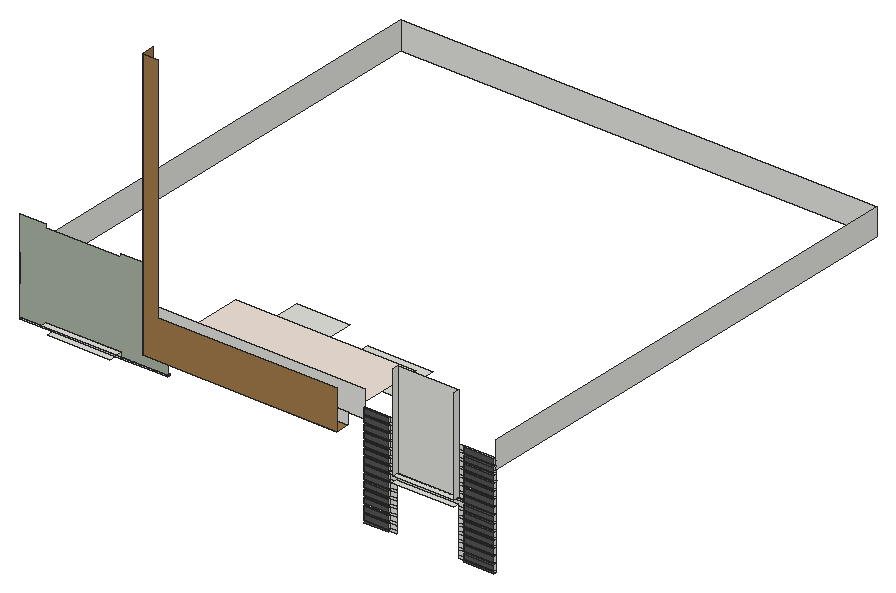
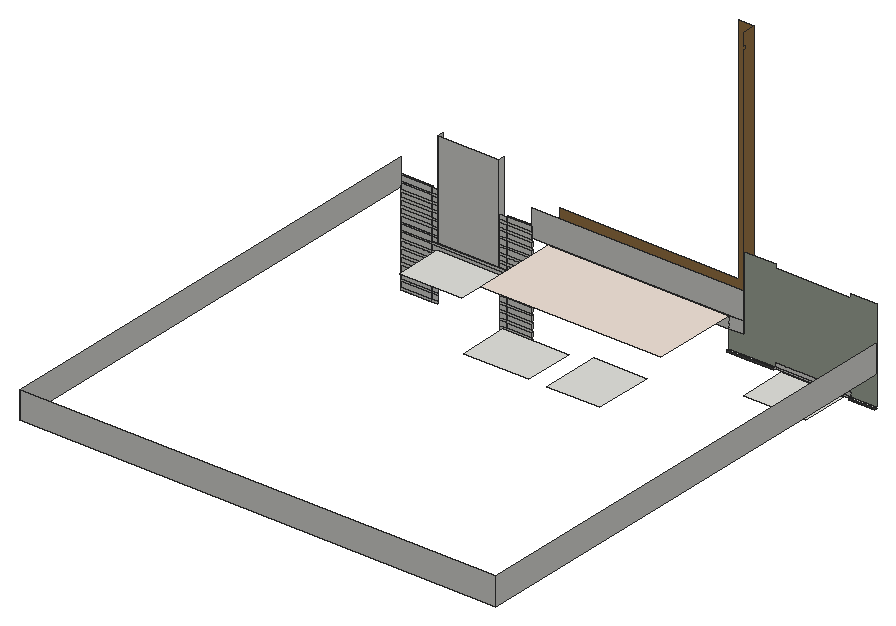
# SketchUp Ruby script. Lengths in inches.
U = 1.inch
M = Sketchup.active_model
def pt(a) = Geom::Point3d.new(a.map { |v| v * U })
def face(e, loops, mat)
  f = e.add_face(loops[0].map { |a| pt(a) })
  loops[1..].each { |l| e.add_face(l.map { |a| pt(a) }).erase! }
  f.material = f.back_material = mat if mat
  f
end
# faces: each face lists its corners as indices into pts; further lists are holes
def faces(e, pts, list, mat = nil) = list.each { |f| face(e, (f[0].is_a?(Array) ? f : [f]).map { |l| l.map { |i| pts[i] } }, mat) }
# xy, xz, yz: faces in a plane at the given z, y or x. An outline is a flat list of corners, or four numbers for a rectangle; further outlines are holes
def ring(l) = l.size == 4 ? [[l[0], l[1]], [l[2], l[1]], [l[2], l[3]], [l[0], l[3]]] : l.each_slice(2).to_a
def flat(e, list, mat, &to3) = list.each { |f| face(e, (f[0].is_a?(Array) ? f : [f]).map { |l| ring(l).map { |u, v| to3.(u, v) } }, mat) }
def xy(e, z, list, mat = nil) = flat(e, list, mat) { |x, y| [x, y, z] }
def xz(e, y, list, mat = nil) = flat(e, list, mat) { |x, z| [x, y, z] }
def yz(e, x, list, mat = nil) = flat(e, list, mat) { |y, z| [x, y, z] }
def lines(e, pts, list) = list.each { |a, b| e.add_line(pt(pts[a]), pt(pts[b])) }
# prism: a flat outline (further loops are holes) pulled along v
def prism(e, loops, v, mat = nil)
  f = face(e, loops, mat); d = Geom::Vector3d.new(v.map { |x| x * U })
  f.pushpull(f.normal.samedirection?(d) ? d.length : -d.length)
end
def box(e, o, s, mat = nil) = prism(e, [[o, [o[0] + s[0], o[1], o[2]], [o[0] + s[0], o[1] + s[1], o[2]], [o[0], o[1] + s[1], o[2]]]], [0, 0, s[2]], mat)
def at(x, y, z, deg = 0) = Geom::Transformation.translation(pt([x, y, z])) * Geom::Transformation.rotation(ORIGIN, Z_AXIS, deg.degrees)
def axes(o, x, y, z) = Geom::Transformation.new([*x, 0, *y, 0, *z, 0, *pt(o).to_a, 1])
def part(name) = M.definitions.add(name)
# library, detail: a bought-in or finely detailed component or shape, given as its bounding box
def library(name, o, s) = part(name).tap { |d| box(d.entities, o, s) }
def detail(e, o, s) = box(e.add_group.entities, o, s)
def put(e, d, t, mat = nil) = e.add_instance(d, t).tap { |i| i.material = mat if mat }
def group(e, t, mat = nil) = e.add_group.tap { |g| g.transformation = t; g.material = mat if mat }.entities
root = M.entities
M.materials.add("Generic\#1").color = [85, 85, 85]
M.materials.add("Generic\#2").color = [170, 178, 163]
M.materials.add("Generic\#3").color = [162, 123, 74]
M.materials.add("Generic\#4").color = [241, 227, 216]
xy(root,660.3125,[[395.4375,28.5,423.8125,31.0625],[508.98,28.5,543.6875,31.0625]],"Generic\#1")
xy(root,663.125,[[395.4375,28.5,423.8125,31.0625],[508.98,28.5,543.6875,31.0625]],"Generic\#1")
xy(root,668.625,[[395.4375,28.5,423.8125,31.0625],[508.98,28.5,543.6875,31.0625]],"Generic\#1")
xy(root,671.4375,[[395.4375,28.5,423.8125,31.0625],[508.98,28.5,543.6875,31.0625]],"Generic\#1")
xy(root,676.9375,[[395.4375,28.5,423.8125,31.0625],[508.98,28.5,543.6875,31.0625]],"Generic\#1")
xy(root,679.75,[[395.4375,28.5,423.8125,31.0625],[508.98,28.5,543.6875,31.0625]],"Generic\#1")
xy(root,685.25,[[395.4375,28.5,423.8125,31.0625],[508.98,28.5,543.6875,31.0625]],"Generic\#1")
xy(root,688.0625,[[395.4375,28.5,423.8125,31.0625],[508.98,28.5,543.6875,31.0625]],"Generic\#1")
xy(root,693.5625,[[395.4375,28.5,423.8125,31.0625],[508.98,28.5,543.6875,31.0625]],"Generic\#1")
xy(root,696.375,[[395.4375,28.5,423.8125,31.0625],[508.98,28.5,543.6875,31.0625]],"Generic\#1")
xy(root,701.875,[[395.4375,28.5,423.8125,31.0625],[508.98,28.5,543.6875,31.0625]],"Generic\#1")
xy(root,704.6875,[[395.4375,28.5,423.8125,31.0625],[508.98,28.5,543.6875,31.0625]],"Generic\#1")
xy(root,710.1875,[[395.4375,28.5,423.8125,31.0625],[508.98,28.5,543.6875,31.0625]],"Generic\#1")
xy(root,713,[[395.4375,28.5,423.8125,31.0625],[508.98,28.5,543.6875,31.0625]],"Generic\#1")
xy(root,715.02,[[430.99,24.0625,501.8,31.0625],[430.99,31.0625,501.8,85.4375]])
xy(root,718.5,[[395.4375,28.5,423.8125,31.0625],[508.98,28.5,543.6875,31.0625]],"Generic\#1")
xy(root,721.3125,[[395.4375,28.5,423.8125,31.0625],[508.98,28.5,543.6875,31.0625]],"Generic\#1")
xy(root,722.19,[[431.91,24.0625,501.98,31.0625]])
xy(root,726.8125,[[395.4375,28.5,423.8125,31.0625],[508.98,28.5,543.6875,31.0625]],"Generic\#1")
xy(root,728.2,[[40.36,24.0625,111.18,31.0625],[40.36,31.0625,111.18,85.4375]])
xy(root,728.625,[[3.6875,31.0625,33.1875,32.9375],[118.35,31.0625,154.5,32.9375],[154.5,31.0625,171.6875,32.9375]])
xy(root,729.625,[[395.4375,28.5,423.8125,31.0625],[508.98,28.5,543.6875,31.0625]],"Generic\#1")
xy(root,730.04,[[275.98,127,350.54,183.625]])
xy(root,730.625,[[3.6875,31.0625,33.1875,32.9375],[118.35,31.0625,154.5,32.9375],[154.5,31.0625,171.6875,32.9375]])
xy(root,735.125,[[395.4375,28.5,423.8125,31.0625],[508.98,28.5,543.6875,31.0625]],"Generic\#1")
xy(root,735.38,[[33.1875,24.0625,118.35,31.0625]])
xy(root,737.0625,[[187.38,127,247.51,193.75]])
xy(root,737.9375,[[395.4375,28.5,423.8125,31.0625],[508.98,28.5,543.6875,31.0625]],"Generic\#1")
xy(root,743.4375,[[395.4375,28.5,423.8125,31.0625],[508.98,28.5,543.6875,31.0625]],"Generic\#1")
xy(root,746.25,[[395.4375,28.5,423.8125,31.0625],[508.98,28.5,543.6875,31.0625]],"Generic\#1")
xy(root,751.4375,[[154.5,15.8125,375.6875,31.0625]],"Generic\#3")
xy(root,751.75,[[395.4375,28.5,423.8125,31.0625],[508.98,28.5,543.6875,31.0625]],"Generic\#1")
xy(root,754.5625,[[395.4375,28.5,423.8125,31.0625],[508.98,28.5,543.6875,31.0625]],"Generic\#1")
xy(root,760.0625,[[395.4375,28.5,423.8125,31.0625],[508.98,28.5,543.6875,31.0625]],"Generic\#1")
xy(root,762.875,[[395.4375,28.5,423.8125,31.0625],[508.98,28.5,543.6875,31.0625]],"Generic\#1")
xy(root,764.625,[[171.6875,31.0625,375.6875,127]],"Generic\#4")
xy(root,768.375,[[395.4375,28.5,423.8125,31.0625],[508.98,28.5,543.6875,31.0625]],"Generic\#1")
xy(root,771.1875,[[395.4375,28.5,423.8125,31.0625],[508.98,28.5,543.6875,31.0625]],"Generic\#1")
xz(root,15.8125,[[154.5,751.4375,375.6875,751.4375,375.6875,795.5,171.6875,795.5,171.6875,1058.1875,154.5,1058.1875]],"Generic\#3")
xz(root,28.5,[[395.4375,663.125,423.8125,668.625],[508.98,663.125,543.6875,668.625],[395.4375,671.4375,423.8125,676.9375],[508.98,671.4375,543.6875,676.9375],[395.4375,679.75,423.8125,685.25],
  [508.98,679.75,543.6875,685.25],[395.4375,688.0625,423.8125,693.5625],[508.98,688.0625,543.6875,693.5625],[395.4375,696.375,423.8125,701.875],[508.98,696.375,543.6875,701.875],
  [395.4375,704.6875,423.8125,710.1875],[508.98,704.6875,543.6875,710.1875],[395.4375,713,423.8125,718.5],[508.98,713,543.6875,718.5],[395.4375,721.3125,423.8125,726.8125],
  [508.98,721.3125,543.6875,726.8125],[395.4375,729.625,423.8125,735.125],[508.98,729.625,543.6875,735.125],[395.4375,737.9375,423.8125,743.4375],[508.98,737.9375,543.6875,743.4375],
  [395.4375,746.25,423.8125,751.75],[508.98,746.25,543.6875,751.75],[395.4375,754.5625,423.8125,760.0625],[508.98,754.5625,543.6875,760.0625],[395.4375,762.875,423.8125,768.375],
  [508.98,762.875,543.6875,768.375],[395.4375,771.1875,423.8125,776.6875],[508.98,771.1875,543.6875,776.6875]],"Generic\#1")
xz(root,31.0625,[[395.4375,660.3125,423.8125,663.125],[423.8125,660.3125,430.99,663.125],[501.8,660.3125,508.98,663.125],[508.98,660.3125,543.6875,663.125],[395.4375,663.125,423.8125,668.625],
  [423.8125,663.125,430.99,668.625],[501.8,663.125,508.98,668.625],[508.98,663.125,543.6875,668.625],[395.4375,668.625,423.8125,671.4375],[423.8125,668.625,430.99,671.4375],
  [501.8,668.625,508.98,671.4375],[508.98,668.625,543.6875,671.4375],[395.4375,671.4375,423.8125,676.9375],[423.8125,671.4375,430.99,676.9375],[501.8,671.4375,508.98,676.9375],
  [508.98,671.4375,543.6875,676.9375],[395.4375,676.9375,423.8125,679.75],[423.8125,676.9375,430.99,679.75],[501.8,676.9375,508.98,679.75],[508.98,676.9375,543.6875,679.75],
  [395.4375,679.75,423.8125,685.25],[423.8125,679.75,430.99,685.25],[501.8,679.75,508.98,685.25],[508.98,679.75,543.6875,685.25],[395.4375,685.25,423.8125,688.0625],
  [423.8125,685.25,430.99,688.0625],[501.8,685.25,508.98,688.0625],[508.98,685.25,543.6875,688.0625],[395.4375,688.0625,423.8125,693.5625],[423.8125,688.0625,430.99,693.5625],
  [501.8,688.0625,508.98,693.5625],[508.98,688.0625,543.6875,693.5625],[395.4375,693.5625,423.8125,696.375],[423.8125,693.5625,430.99,696.375],[501.8,693.5625,508.98,696.375],
  [508.98,693.5625,543.6875,696.375],[395.4375,696.375,423.8125,701.875],[423.8125,696.375,430.99,701.875],[501.8,696.375,508.98,701.875],[508.98,696.375,543.6875,701.875],
  [395.4375,701.875,423.8125,704.6875],[423.8125,701.875,430.99,704.6875],[501.8,701.875,508.98,704.6875],[508.98,701.875,543.6875,704.6875],[395.4375,704.6875,423.8125,710.1875],
  [423.8125,704.6875,430.99,710.1875],[501.8,704.6875,508.98,710.1875],[508.98,704.6875,543.6875,710.1875],[395.4375,710.1875,423.8125,713],[423.8125,710.1875,430.99,713],
  [501.8,710.1875,508.98,713],[508.98,710.1875,543.6875,713],[395.4375,713,423.8125,718.5],[423.8125,713,430.99,713,430.99,715.02,501.8,715.02,501.8,713,508.98,713,508.98,718.5,423.8125,718.5],[508.98,713,543.6875,718.5],
  [395.4375,718.5,423.8125,721.3125],[423.8125,718.5,508.98,721.3125],[508.98,718.5,543.6875,721.3125],[395.4375,721.3125,423.8125,726.8125],[423.8125,721.3125,508.98,722.19],
  [508.98,721.3125,543.6875,726.8125],[423.8125,722.19,431.91,726.8125],[431.91,722.19,501.98,831.53],[501.98,722.19,508.98,726.8125],[395.4375,726.8125,423.8125,729.625],
  [423.8125,726.8125,431.91,729.625],[501.98,726.8125,508.98,729.625],[508.98,726.8125,543.6875,729.625],[33.1875,728.625,118.35,730.625],[395.4375,729.625,423.8125,735.125],
  [423.8125,729.625,431.91,735.125],[501.98,729.625,508.98,735.125],[508.98,729.625,543.6875,735.125],[33.1875,730.625,118.35,735.38],[395.4375,735.125,423.8125,737.9375],
  [423.8125,735.125,431.91,737.9375],[501.98,735.125,508.98,737.9375],[508.98,735.125,543.6875,737.9375],[395.4375,737.9375,423.8125,743.4375],[423.8125,737.9375,431.91,743.4375],
  [501.98,737.9375,508.98,743.4375],[508.98,737.9375,543.6875,743.4375],[395.4375,743.4375,423.8125,746.25],[423.8125,743.4375,431.91,746.25],[501.98,743.4375,508.98,746.25],
  [508.98,743.4375,543.6875,746.25],[395.4375,746.25,423.8125,751.75],[423.8125,746.25,431.91,751.75],[501.98,746.25,508.98,751.75],[508.98,746.25,543.6875,751.75],
  [154.5,751.4375,171.6875,764.625],[171.6875,751.4375,375.6875,764.625],[395.4375,751.75,423.8125,754.5625],[423.8125,751.75,431.91,754.5625],[501.98,751.75,508.98,754.5625],
  [508.98,751.75,543.6875,754.5625],[395.4375,754.5625,423.8125,760.0625],[423.8125,754.5625,431.91,760.0625],[501.98,754.5625,508.98,760.0625],[508.98,754.5625,543.6875,760.0625],
  [395.4375,760.0625,423.8125,762.875],[423.8125,760.0625,431.91,762.875],[501.98,760.0625,508.98,762.875],[508.98,760.0625,543.6875,762.875],[395.4375,762.875,423.8125,768.375],
  [423.8125,762.875,431.91,768.375],[501.98,762.875,508.98,768.375],[508.98,762.875,543.6875,768.375],[154.5,764.625,395.4375,795.5],[395.4375,768.375,423.8125,771.1875],
  [423.8125,768.375,431.91,771.1875],[501.98,768.375,508.98,771.1875],[508.98,768.375,543.6875,771.1875],[395.4375,771.1875,423.8125,776.6875],[423.8125,771.1875,431.91,776.6875],
  [501.98,771.1875,508.98,776.6875],[508.98,771.1875,543.6875,776.6875]])
xz(root,31.0625,[[3.6875,730.625,33.1875,730.625,33.1875,735.38,118.35,735.38,118.35,730.625,171.6875,730.625,171.6875,751.4375,154.5,751.4375,154.5,835.5,118.35,835.5,118.35,831.53,33.1875,831.53,33.1875,835.5,3.6875,835.5]],"Generic\#2")
xz(root,32.9375,[[3.6875,728.625,33.1875,730.625],[118.35,728.625,171.6875,730.625]],"Generic\#1")
xz(root,571.0625,[[3.6875,764.625,543.6875,795.5]])
yz(root,3.6875,[[31.0625,764.625,571.0625,795.5]])
yz(root,33.1875,[[31.0625,728.625,32.9375,730.625]])
yz(root,118.35,[[31.0625,728.625,32.9375,730.625]])
yz(root,154.5,[[15.8125,751.4375,15.8125,1058.1875,31.0625,1058.1875,31.0625,1044.8125,27.375,1044.8125,27.375,1040.6875,31.0625,1040.6875,31.0625,751.4375]],"Generic\#3")
yz(root,395.4375,[[28.5,663.125,31.0625,668.625],[28.5,671.4375,31.0625,676.9375],[28.5,679.75,31.0625,685.25],[28.5,688.0625,31.0625,693.5625],[28.5,696.375,31.0625,701.875],
  [28.5,704.6875,31.0625,710.1875],[28.5,713,31.0625,718.5],[28.5,721.3125,31.0625,726.8125],[28.5,729.625,31.0625,735.125],[28.5,737.9375,31.0625,743.4375],
  [28.5,746.25,31.0625,751.75],[28.5,754.5625,31.0625,760.0625],[28.5,762.875,31.0625,764.625],[28.5,764.625,31.0625,768.375],[28.5,771.1875,31.0625,776.6875]])
yz(root,423.8125,[[28.5,663.125,31.0625,668.625],[28.5,671.4375,31.0625,676.9375],[28.5,679.75,31.0625,685.25],[28.5,688.0625,31.0625,693.5625],[28.5,696.375,31.0625,701.875],
  [28.5,704.6875,31.0625,710.1875],[28.5,713,31.0625,718.5],[28.5,721.3125,31.0625,722.19],[28.5,722.19,31.0625,726.8125],[28.5,729.625,31.0625,735.125],
  [28.5,737.9375,31.0625,743.4375],[28.5,746.25,31.0625,751.75],[28.5,754.5625,31.0625,760.0625],[28.5,762.875,31.0625,768.375],[28.5,771.1875,31.0625,776.6875]])
yz(root,431.91,[[24.0625,722.19,31.0625,831.53]])
yz(root,501.98,[[24.0625,722.19,31.0625,831.53]])
yz(root,508.98,[[28.5,663.125,31.0625,668.625],[28.5,671.4375,31.0625,676.9375],[28.5,679.75,31.0625,685.25],[28.5,688.0625,31.0625,693.5625],[28.5,696.375,31.0625,701.875],
  [28.5,704.6875,31.0625,710.1875],[28.5,713,31.0625,718.5],[28.5,721.3125,31.0625,722.19],[28.5,722.19,31.0625,726.8125],[28.5,729.625,31.0625,735.125],
  [28.5,737.9375,31.0625,743.4375],[28.5,746.25,31.0625,751.75],[28.5,754.5625,31.0625,760.0625],[28.5,762.875,31.0625,768.375],[28.5,771.1875,31.0625,776.6875]])
yz(root,543.6875,[[28.5,663.125,31.0625,668.625],[28.5,671.4375,31.0625,676.9375],[28.5,679.75,31.0625,685.25],[28.5,688.0625,31.0625,693.5625],[28.5,696.375,31.0625,701.875],
  [28.5,704.6875,31.0625,710.1875],[28.5,713,31.0625,718.5],[28.5,721.3125,31.0625,726.8125],[28.5,729.625,31.0625,735.125],[28.5,737.9375,31.0625,743.4375],
  [28.5,746.25,31.0625,751.75],[28.5,754.5625,31.0625,760.0625],[28.5,762.875,31.0625,764.625],[28.5,764.625,31.0625,768.375],[31.0625,764.625,571.0625,795.5],
  [28.5,771.1875,31.0625,776.6875]])
